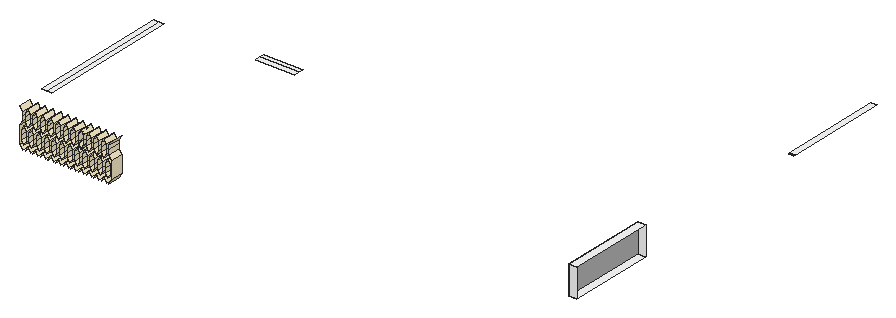
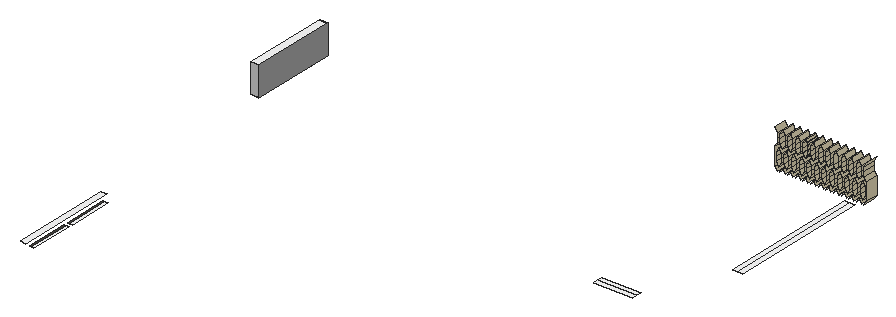
# SketchUp Ruby script. Lengths in inches.
U = 1.inch
M = Sketchup.active_model
def pt(a) = Geom::Point3d.new(a.map { |v| v * U })
def face(e, loops, mat)
  f = e.add_face(loops[0].map { |a| pt(a) })
  loops[1..].each { |l| e.add_face(l.map { |a| pt(a) }).erase! }
  f.material = f.back_material = mat if mat
  f
end
# faces: each face lists its corners as indices into pts; further lists are holes
def faces(e, pts, list, mat = nil) = list.each { |f| face(e, (f[0].is_a?(Array) ? f : [f]).map { |l| l.map { |i| pts[i] } }, mat) }
# xy, xz, yz: faces in a plane at the given z, y or x. An outline is a flat list of corners, or four numbers for a rectangle; further outlines are holes
def ring(l) = l.size == 4 ? [[l[0], l[1]], [l[2], l[1]], [l[2], l[3]], [l[0], l[3]]] : l.each_slice(2).to_a
def flat(e, list, mat, &to3) = list.each { |f| face(e, (f[0].is_a?(Array) ? f : [f]).map { |l| ring(l).map { |u, v| to3.(u, v) } }, mat) }
def xy(e, z, list, mat = nil) = flat(e, list, mat) { |x, y| [x, y, z] }
def xz(e, y, list, mat = nil) = flat(e, list, mat) { |x, z| [x, y, z] }
def yz(e, x, list, mat = nil) = flat(e, list, mat) { |y, z| [x, y, z] }
def lines(e, pts, list) = list.each { |a, b| e.add_line(pt(pts[a]), pt(pts[b])) }
# prism: a flat outline (further loops are holes) pulled along v
def prism(e, loops, v, mat = nil)
  f = face(e, loops, mat); d = Geom::Vector3d.new(v.map { |x| x * U })
  f.pushpull(f.normal.samedirection?(d) ? d.length : -d.length)
end
def box(e, o, s, mat = nil) = prism(e, [[o, [o[0] + s[0], o[1], o[2]], [o[0] + s[0], o[1] + s[1], o[2]], [o[0], o[1] + s[1], o[2]]]], [0, 0, s[2]], mat)
def at(x, y, z, deg = 0) = Geom::Transformation.translation(pt([x, y, z])) * Geom::Transformation.rotation(ORIGIN, Z_AXIS, deg.degrees)
def axes(o, x, y, z) = Geom::Transformation.new([*x, 0, *y, 0, *z, 0, *pt(o).to_a, 1])
def part(name) = M.definitions.add(name)
# library, detail: a bought-in or finely detailed component or shape, given as its bounding box
def library(name, o, s) = part(name).tap { |d| box(d.entities, o, s) }
def detail(e, o, s) = box(e.add_group.entities, o, s)
def put(e, d, t, mat = nil) = e.add_instance(d, t).tap { |i| i.material = mat if mat }
def group(e, t, mat = nil) = e.add_group.tap { |g| g.transformation = t; g.material = mat if mat }.entities
root = M.entities
M.materials.add("D01_Frost_White").color = [255, 242, 206]
M.materials.add("Glass_Mirror_01").color = [185, 185, 185]
M.materials.add("M00_Soft_Cloud").color = [255, 255, 255]
M.materials.add("Wood_Planks_01_1K").color = [69, 67, 63]
xy(root,220.1287,[[555,437.068,557.1509,475.3136],[555,479.3136,557.1509,517.5592]],"M00_Soft_Cloud")
xy(root,220.1287,[[557.1509,437.068,559.3018,475.3136],[557.1509,479.3136,559.3018,517.5592]],"Wood_Planks_01_1K")
xy(root,221.934,[[189.7692,309,223.7462,313.5],[189.7692,313.5,223.7462,318]],"M00_Soft_Cloud")
xy(root,222.3305,[[564,184.6361,571,259.8187]],"M00_Soft_Cloud")
xy(root,224.1287,[[559.3018,433.068,564,521.5592]],"M00_Soft_Cloud")
xy(root,242.0154,[[196.5333,109.0676,196.5333,109.0676,196.5333,119.6039,196.5333,119.6039]],"D01_Frost_White")
xy(root,245.0192,[[126,153.6841,130.5,276.2837],[130.5,153.6841,135,276.2837]],"M00_Soft_Cloud")
xy(root,247.6528,[[564,184.6361,571,259.8187]],"M00_Soft_Cloud")
xy(root,253.2819,[[194.3471,109.0676,194.3471,109.0676,194.3471,119.6039,194.3471,119.6039]],"D01_Frost_White")
xz(root,109.0676,[[209.933,226.9934,209.933,227.0116,209.9276,227.0025],[196.5368,242.0094,196.5404,242.0154,196.5368,242.0215,196.5333,242.0154],[209.933,242.0094,209.933,242.0154,209.9312,242.0124],[183.1639,242.0124,183.1675,242.0185,183.1639,242.0245],[196.5333,242.0154,196.5333,242.0154,196.5261,242.0276],
  [196.5333,242.0154,196.5368,242.0215,196.5297,242.0336,196.5261,242.0276],[196.5404,242.0154,198.7337,245.7225,196.5368,242.0215],[196.5368,242.0215,198.7337,245.7225,196.5297,242.0336],[169.7802,242.0276,167.5797,245.7709,167.5797,245.7831],[196.5261,242.0276,195.801,243.2733,195.4366,243.8932],
  [196.5261,242.0276,196.0916,242.7789,195.801,243.2733],[196.5261,242.0276,196.5297,242.0336,196.0916,242.7789],[196.0916,242.7789,194.3399,245.8073,194.3399,245.783,195.801,243.2733],[195.4366,243.8932,194.3399,245.7709,194.3399,245.7588],[198.7337,245.7225,198.7409,245.7345,198.7409,245.7345],
  [198.7337,245.7225,198.7409,245.7345,198.7516,253.203],[198.7409,245.7345,198.7409,245.7345,198.7444,245.7406],[198.7409,245.7345,198.7444,245.7406,198.7516,253.203],[198.7444,245.7406,198.7552,245.7588,198.7552,253.2576,196.5547,257.001,196.5618,256.9888,198.7516,253.2394,198.7516,253.203],[194.3399,245.7709,194.3399,245.783,194.3364,245.7891,194.3363,245.777],
  [194.3399,245.783,194.3399,245.8073,194.3364,245.8134,194.3364,245.7891],[167.5797,245.7831,167.5797,253.2698,167.5833,253.2759],[194.3364,245.7891,194.3364,245.8134,194.3363,245.7892],[194.3399,245.8073,194.3399,247.2979,194.3364,245.8134],[194.3364,245.8134,194.3399,247.2979,194.3399,248.2868],
  [194.3364,245.8134,194.3399,248.2868,194.3399,249.5264],[194.3399,247.2979,194.3542,253.2819,194.347,253.2698,194.3435,253.2637,194.3435,253.2759,194.3471,253.2819,194.347,253.2698,194.3399,248.2868],[194.3399,249.5264,194.3435,253.2637,194.3399,253.2576],[198.7516,253.203,198.7516,253.2273,196.5618,256.9888],[198.7516,253.203,198.7516,253.2273,198.7516,253.2273],
  [198.7516,253.2273,198.7516,253.2394,196.5618,256.9888],[194.3435,253.2637,194.347,253.2698,194.3471,253.2819,194.3435,253.2759],[194.347,253.2698,194.3542,253.2819,194.3542,253.294,194.3471,253.2819],[194.3471,253.2819,194.3471,253.2819,194.3542,253.294],[194.3542,253.2819,194.7923,254.0272,194.3542,253.294],
  [194.3542,253.294,194.7923,254.0272,195.0829,254.5216],[194.3542,253.294,195.0829,254.5216,195.4473,255.1415],[194.7923,254.0272,196.5618,256.9888,196.5547,257.001,195.0829,254.5216],[195.0829,254.5216,196.5547,257.001,196.5529,257.004,196.5493,257.004,195.4473,255.1415],[195.4473,255.1415,196.5493,257.004,196.5422,257.004]],"D01_Frost_White")
xz(root,184.6361,[[564,222.3305,571,247.6528]],"M00_Soft_Cloud")
xz(root,259.8187,[[564,222.3305,571,247.6528]],"M00_Soft_Cloud")
yz(root,143.0236,[[109.0676,227.0238,119.6039,242.0215]],"D01_Frost_White")
yz(root,144.165,[[109.0676,230.7732,119.6039,234.5226],[109.0676,234.5226,119.6039,238.2721]],"D01_Frost_White")
yz(root,145.2277,[[109.0676,245.7709,119.6039,249.5204],[109.0676,249.5204,119.6039,253.2698]],"D01_Frost_White")
yz(root,147.5105,[[109.0676,245.7709,119.6039,249.5204],[109.0676,249.5204,119.6039,253.2698]],"D01_Frost_White")
yz(root,148.5731,[[109.0676,230.7732,119.6039,234.5226],[109.0676,234.5226,119.6039,238.2721]],"D01_Frost_White")
yz(root,150.856,[[109.0676,230.7732,119.6039,234.5226],[109.0676,234.5226,119.6039,238.2721]],"D01_Frost_White")
yz(root,151.9186,[[109.0676,245.7709,119.6039,249.5204],[109.0676,249.5204,119.6039,253.2698]],"D01_Frost_White")
yz(root,154.2015,[[109.0676,245.7709,119.6039,249.5204],[109.0676,249.5204,119.6039,253.2698]],"D01_Frost_White")
yz(root,155.2641,[[109.0676,230.7732,119.6039,234.5226],[109.0676,234.5226,119.6039,238.2721]],"D01_Frost_White")
yz(root,157.5433,[[109.0676,230.7732,119.6039,234.5226],[109.0676,234.5226,119.6039,238.2721]],"D01_Frost_White")
yz(root,158.606,[[109.0676,245.7709,119.6039,249.5204],[109.0676,249.5204,119.6039,253.2698]],"D01_Frost_White")
yz(root,160.8888,[[109.0676,245.7709,119.6039,249.5204],[109.0676,249.5204,119.6039,253.2698]],"D01_Frost_White")
yz(root,161.9514,[[109.0676,230.7732,119.6039,234.5226],[109.0676,234.5226,119.6039,238.2721]],"D01_Frost_White")
yz(root,164.2343,[[109.0676,230.7732,119.6039,234.5226],[109.0676,234.5226,119.6039,238.2721]],"D01_Frost_White")
yz(root,165.2969,[[109.0676,245.7709,119.6039,249.5204],[109.0676,249.5204,119.6039,253.2698]],"D01_Frost_White")
yz(root,167.5797,[[109.0676,245.7709,119.6039,245.7831],[109.0676,245.7831,119.6039,249.5204],[109.0676,249.5204,119.6039,253.2698]],"D01_Frost_White")
yz(root,168.6424,[[109.0676,230.7732,119.6039,234.5226],[109.0676,234.5226,119.6039,238.2721]],"D01_Frost_White")
yz(root,170.9288,[[109.0676,230.7671,119.6039,234.5166],[109.0676,234.5166,119.6039,238.266]],"D01_Frost_White")
yz(root,174.2743,[[109.0676,245.7649,119.6039,249.5143],[109.0676,249.5143,119.6039,253.2637]],"D01_Frost_White")
yz(root,175.3369,[[109.0676,230.7671,119.6039,234.5166],[109.0676,234.5166,119.6039,238.266]],"D01_Frost_White")
yz(root,177.6197,[[109.0676,230.7671,119.6039,234.5166],[109.0676,234.5166,119.6039,238.266]],"D01_Frost_White")
yz(root,178.6824,[[109.0676,245.7649,119.6039,249.5143],[109.0676,249.5143,119.6039,253.2637]],"D01_Frost_White")
yz(root,180.9652,[[109.0676,245.7649,119.6039,249.5143],[109.0676,249.5143,119.6039,253.2637]],"D01_Frost_White")
yz(root,182.0278,[[109.0676,230.7671,119.6039,234.5166],[109.0676,234.5166,119.6039,238.266]],"D01_Frost_White")
yz(root,183.1639,[[109.0676,242.0124,119.6039,242.0245]],"D01_Frost_White")
yz(root,184.3035,[[109.0676,230.7611,119.6039,234.5105],[109.0676,234.5105,119.6039,238.2599]],"D01_Frost_White")
yz(root,185.3661,[[109.0676,245.7588,119.6039,249.5082],[109.0676,249.5082,119.6039,253.2576]],"D01_Frost_White")
yz(root,187.649,[[109.0676,245.7588,119.6039,249.5082],[109.0676,249.5082,119.6039,253.2576]],"D01_Frost_White")
yz(root,188.7116,[[109.0676,230.7611,119.6039,234.5105],[109.0676,234.5105,119.6039,238.2599]],"D01_Frost_White")
yz(root,190.9945,[[109.0676,230.7611,119.6039,234.5105],[109.0676,234.5105,119.6039,238.2599]],"D01_Frost_White")
yz(root,192.0571,[[109.0676,245.7588,119.6039,249.5082],[109.0676,249.5082,119.6039,253.2576]],"D01_Frost_White")
yz(root,194.3399,[[109.0676,245.7588,119.6039,245.7709],[109.0676,245.7709,119.6039,245.783],[109.0676,245.783,119.6039,245.8073],[109.0676,247.2979,119.6039,248.2868],[109.0676,248.2868,119.6039,249.5082],
  [109.0676,249.5082,119.6039,249.5264],[109.0676,249.5264,119.6039,253.2576]],"D01_Frost_White")
yz(root,194.3435,[[109.0676,253.2637,119.6039,253.2759]],"D01_Frost_White")
yz(root,194.3542,[[109.0676,253.2819,119.6039,253.294]],"D01_Frost_White")
yz(root,195.4025,[[109.0676,230.7611,119.6039,234.5105],[109.0676,234.5105,119.6039,238.2599]],"D01_Frost_White")
yz(root,197.6925,[[109.0676,230.7611,119.6039,234.5105],[109.0676,234.5105,119.6039,238.2599]],"D01_Frost_White")
yz(root,198.7552,[[109.0676,245.7588,119.6039,249.5082],[109.0676,249.5082,119.6039,253.2576]],"D01_Frost_White")
yz(root,201.038,[[109.0676,245.7588,119.6039,249.5082],[109.0676,249.5082,119.6039,253.2576]],"D01_Frost_White")
yz(root,202.1006,[[109.0676,230.7611,119.6039,234.5105],[109.0676,234.5105,119.6039,238.2599]],"D01_Frost_White")
yz(root,204.3835,[[109.0676,230.7611,119.6039,234.5105],[109.0676,234.5105,119.6039,238.2599]],"D01_Frost_White")
yz(root,205.4461,[[109.0676,245.7588,119.6039,249.5082],[109.0676,249.5082,119.6039,253.2576]],"D01_Frost_White")
yz(root,207.7289,[[109.0676,245.7588,119.6039,249.5082],[109.0676,249.5082,119.6039,253.2576]],"D01_Frost_White")
yz(root,208.7916,[[109.0676,230.7611,119.6039,234.5105],[109.0676,234.5105,119.6039,238.2599]],"D01_Frost_White")
yz(root,209.933,[[109.0676,226.9934,119.6039,227.0116],[109.0676,242.0094,119.6039,242.0154]],"D01_Frost_White")
yz(root,211.0673,[[109.0676,230.755,119.6039,234.5044],[109.0676,234.5044,119.6039,238.2539]],"D01_Frost_White")
yz(root,212.1299,[[109.0676,245.7527,119.6039,249.5021],[109.0676,249.5021,119.6039,253.2516]],"D01_Frost_White")
yz(root,214.4127,[[109.0676,245.7527,119.6039,249.5021],[109.0676,249.5021,119.6039,253.2516]],"D01_Frost_White")
yz(root,215.4754,[[109.0676,230.755,119.6039,234.5044],[109.0676,234.5044,119.6039,238.2539]],"D01_Frost_White")
yz(root,217.7582,[[109.0676,230.755,119.6039,234.5044],[109.0676,234.5044,119.6039,238.2539]],"D01_Frost_White")
yz(root,218.8208,[[109.0676,245.7527,119.6039,249.5021],[109.0676,249.5021,119.6039,253.2516]],"D01_Frost_White")
yz(root,221.1037,[[109.0676,245.7527,119.6039,249.5021],[109.0676,249.5021,119.6039,253.2516]],"D01_Frost_White")
yz(root,222.1663,[[109.0676,230.755,119.6039,234.5044],[109.0676,234.5044,119.6039,238.2539]],"D01_Frost_White")
yz(root,223.3077,[[109.0676,227.0056,119.6039,242.0033]],"D01_Frost_White")
yz(root,564,[[184.6361,222.3305,259.8187,247.6528]],"Glass_Mirror_01")
p = [[143.0236,109.0676,227.0238],[145.2277,109.0676,223.2743],[145.2277,119.6039,223.2743],[143.0236,119.6039,227.0238],[147.5105,109.0676,223.2743],[149.7146,109.0676,227.0238],
  [149.7146,119.6039,227.0238],[147.5105,119.6039,223.2743],[151.9186,109.0676,223.2743],[151.9186,119.6039,223.2743],[154.2015,109.0676,223.2743],[156.4037,109.0676,227.0207],
  [156.4037,119.6039,227.0207],[154.2015,119.6039,223.2743],[158.606,109.0676,223.2743],[158.606,119.6039,223.2743],[160.8888,109.0676,223.2743],[163.0929,109.0676,227.0238],
  [163.0929,119.6039,227.0238],[160.8888,119.6039,223.2743],[165.2969,109.0676,223.2743],[165.2969,119.6039,223.2743],[167.5797,109.0676,223.2743],[167.5833,109.0676,223.2804],
  [167.5833,119.6039,223.2804],[167.5797,119.6039,223.2743],[169.7874,109.0676,227.0177],[169.7874,119.6039,227.0177],[171.9878,109.0676,223.2622],[171.9878,119.6039,223.2622],
  [174.2743,109.0676,223.2683],[176.4783,109.0676,227.0177],[176.4783,119.6039,227.0177],[174.2743,119.6039,223.2683],[178.6824,109.0676,223.2683],[178.6824,119.6039,223.2683],
  [180.9652,109.0676,223.2683],[183.1639,109.0676,227.0086],[183.1639,119.6039,227.0086],[180.9652,119.6039,223.2683],[185.3661,109.0676,223.2622],[185.3661,119.6039,223.2622],
  [187.649,109.0676,223.2622],[189.853,109.0676,227.0116],[189.853,119.6039,227.0116],[187.649,119.6039,223.2622],[192.0571,109.0676,223.2622],[192.0571,119.6039,223.2622],
  [194.3399,109.0676,223.2622],[196.544,109.0676,227.0116],[196.544,119.6039,227.0116],[194.3399,119.6039,223.2622],[198.748,109.0676,223.2622],[198.748,119.6039,223.2622],
  [201.038,109.0676,223.2622],[203.242,109.0676,227.0116],[203.242,119.6039,227.0116],[201.038,119.6039,223.2622],[205.4461,109.0676,223.2622],[205.4461,119.6039,223.2622],
  [207.7289,109.0676,223.2622],[209.9276,109.0676,227.0025],[209.9276,119.6039,227.0025],[207.7289,119.6039,223.2622],[209.933,109.0676,226.9934],[212.1299,109.0676,223.2561],
  [212.1299,119.6039,223.2561],[209.933,119.6039,226.9934],[214.4127,109.0676,223.2561],[216.6168,109.0676,227.0056],[216.6168,119.6039,227.0056],[214.4127,119.6039,223.2561],
  [218.8208,109.0676,223.2561],[218.8208,119.6039,223.2561],[221.1037,109.0676,223.2561],[223.3077,109.0676,227.0056],[223.3077,119.6039,227.0056],[221.1037,119.6039,223.2561],
  [146.3691,109.0676,227.0238],[144.165,109.0676,230.7732],[144.165,119.6039,230.7732],[146.3691,119.6039,227.0238],[148.5731,109.0676,230.7732],[148.5731,119.6039,230.7732],
  [153.06,109.0676,227.0238],[150.856,109.0676,230.7732],[150.856,119.6039,230.7732],[153.06,119.6039,227.0238],[155.2641,109.0676,230.7732],[155.2641,119.6039,230.7732],
  [159.7474,109.0676,227.0238],[157.5433,109.0676,230.7732],[157.5433,119.6039,230.7732],[159.7474,119.6039,227.0238],[161.9514,109.0676,230.7732],[161.9514,119.6039,230.7732],
  [166.4383,109.0676,227.0238],[164.2343,109.0676,230.7732],[164.2343,119.6039,230.7732],[166.4383,119.6039,227.0238],[168.6424,109.0676,230.7732],[168.6424,119.6039,230.7732],
  [173.1328,109.0676,227.0177],[170.9288,109.0676,230.7671],[170.9288,119.6039,230.7671],[173.1328,119.6039,227.0177],[175.3369,109.0676,230.7671],[175.3369,119.6039,230.7671],
  [179.8238,109.0676,227.0177],[177.6197,109.0676,230.7671],[177.6197,119.6039,230.7671],[179.8238,119.6039,227.0177],[182.0278,109.0676,230.7671],[182.0278,119.6039,230.7671],
  [186.5076,109.0676,227.0116],[184.3035,109.0676,230.7611],[184.3035,119.6039,230.7611],[186.5076,119.6039,227.0116],[188.7116,109.0676,230.7611],[188.7116,119.6039,230.7611],
  [193.1985,109.0676,227.0116],[190.9945,109.0676,230.7611],[190.9945,119.6039,230.7611],[193.1985,119.6039,227.0116],[195.4025,109.0676,230.7611],[195.4025,119.6039,230.7611],
  [199.8966,109.0676,227.0116],[197.6925,109.0676,230.7611],[197.6925,119.6039,230.7611],[199.8966,119.6039,227.0116],[202.1006,109.0676,230.7611],[202.1006,119.6039,230.7611],
  [206.5875,109.0676,227.0116],[204.3835,109.0676,230.7611],[204.3835,119.6039,230.7611],[206.5875,119.6039,227.0116],[208.7916,109.0676,230.7611],[208.7916,119.6039,230.7611],
  [209.933,109.0676,227.0116],[209.933,119.6039,227.0116],[213.2713,109.0676,227.0056],[211.0673,109.0676,230.755],[211.0673,119.6039,230.755],[213.2713,119.6039,227.0056],
  [215.4754,109.0676,230.755],[215.4754,119.6039,230.755],[219.9622,109.0676,227.0056],[217.7582,109.0676,230.755],[217.7582,119.6039,230.755],[219.9622,119.6039,227.0056],
  [222.1663,109.0676,230.755],[222.1663,119.6039,230.755],[144.165,109.0676,238.2721],[146.3691,109.0676,242.0215],[146.3691,119.6039,242.0215],[144.165,119.6039,238.2721],
  [148.5731,109.0676,238.2721],[148.5731,119.6039,238.2721],[150.856,109.0676,238.2721],[153.06,109.0676,242.0215],[153.06,119.6039,242.0215],[150.856,119.6039,238.2721],
  [155.2641,109.0676,238.2721],[155.2641,119.6039,238.2721],[157.5433,109.0676,238.2721],[159.7474,109.0676,242.0215],[159.7474,119.6039,242.0215],[157.5433,119.6039,238.2721],
  [161.9514,109.0676,238.2721],[161.9514,119.6039,238.2721],[164.2343,109.0676,238.2721],[166.4383,109.0676,242.0215],[166.4383,119.6039,242.0215],[164.2343,119.6039,238.2721],
  [168.6424,109.0676,238.2721],[168.6424,119.6039,238.2721],[170.9288,109.0676,238.266],[173.1328,109.0676,242.0154],[173.1328,119.6039,242.0154],[170.9288,119.6039,238.266],
  [175.3369,109.0676,238.266],[175.3369,119.6039,238.266],[177.6197,109.0676,238.266],[179.8238,109.0676,242.0154],[179.8238,119.6039,242.0154],[177.6197,119.6039,238.266],
  [182.0278,109.0676,238.266],[182.0278,119.6039,238.266],[184.3035,109.0676,238.2599],[186.5076,109.0676,242.0094],[186.5076,119.6039,242.0094],[184.3035,119.6039,238.2599],
  [188.7116,109.0676,238.2599],[188.7116,119.6039,238.2599],[190.9945,109.0676,238.2599],[193.1985,109.0676,242.0094],[193.1985,119.6039,242.0094],[190.9945,119.6039,238.2599],
  [195.4025,109.0676,238.2599],[195.4025,119.6039,238.2599],[197.6925,109.0676,238.2599],[199.8966,109.0676,242.0094],[199.8966,119.6039,242.0094],[197.6925,119.6039,238.2599],
  [202.1006,109.0676,238.2599],[202.1006,119.6039,238.2599],[204.3835,109.0676,238.2599],[206.5875,109.0676,242.0094],[206.5875,119.6039,242.0094],[204.3835,119.6039,238.2599],
  [208.7916,109.0676,238.2599],[208.7916,119.6039,238.2599],[211.0673,109.0676,238.2539],[213.2713,109.0676,242.0033],[213.2713,119.6039,242.0033],[211.0673,119.6039,238.2539],
  [215.4754,109.0676,238.2539],[215.4754,119.6039,238.2539],[217.7582,109.0676,238.2539],[219.9622,109.0676,242.0033],[219.9622,119.6039,242.0033],[217.7582,119.6039,238.2539],
  [222.1663,109.0676,238.2539],[222.1663,119.6039,238.2539],[145.2277,109.0676,245.7709],[143.0236,109.0676,242.0215],[143.0236,119.6039,242.0215],[145.2277,119.6039,245.7709],
  [149.7146,109.0676,242.0215],[147.5105,109.0676,245.7709],[147.5105,119.6039,245.7709],[149.7146,119.6039,242.0215],[151.9186,109.0676,245.7709],[151.9186,119.6039,245.7709],
  [156.4037,109.0676,242.0245],[154.2015,109.0676,245.7709],[154.2015,119.6039,245.7709],[156.4037,119.6039,242.0245],[158.606,109.0676,245.7709],[158.606,119.6039,245.7709],
  [163.0929,109.0676,242.0215],[160.8888,109.0676,245.7709],[160.8888,119.6039,245.7709],[163.0929,119.6039,242.0215],[165.2969,109.0676,245.7709],[165.2969,119.6039,245.7709],
  [169.7802,109.0676,242.0276],[167.5797,109.0676,245.7709],[167.5797,119.6039,245.7709],[169.7802,119.6039,242.0276],[171.9843,109.0676,245.7649],[171.9843,119.6039,245.7649],
  [176.4783,109.0676,242.0154],[174.2743,109.0676,245.7649],[174.2743,119.6039,245.7649],[176.4783,119.6039,242.0154],[178.6824,109.0676,245.7649],[178.6824,119.6039,245.7649],
  [183.1639,109.0676,242.0245],[180.9652,109.0676,245.7649],[180.9652,119.6039,245.7649],[183.1639,119.6039,242.0245],[183.1675,109.0676,242.0185],[183.1639,109.0676,242.0124],
  [183.1639,119.6039,242.0124],[183.1675,119.6039,242.0185],[185.3661,109.0676,245.7588],[185.3661,119.6039,245.7588],[189.853,109.0676,242.0094],[187.649,109.0676,245.7588],
  [187.649,119.6039,245.7588],[189.853,119.6039,242.0094],[192.0571,109.0676,245.7588],[192.0571,119.6039,245.7588],[196.5261,109.0676,242.0276],[195.4366,109.0676,243.8932],
  [195.4366,119.6039,243.8932],[196.5261,119.6039,242.0276],[196.5404,109.0676,242.0154],[196.5368,109.0676,242.0094],[196.5368,119.6039,242.0094],[196.5404,119.6039,242.0154],
  [196.5333,109.0676,242.0154],[196.5333,119.6039,242.0154],[196.5368,109.0676,242.0215],[196.5368,119.6039,242.0215],[196.5333,109.0676,242.0154],[196.5333,119.6039,242.0154],
  [198.7337,109.0676,245.7225],[198.7337,119.6039,245.7225],[203.242,109.0676,242.0094],[201.038,109.0676,245.7588],[201.038,119.6039,245.7588],[203.242,119.6039,242.0094],
  [205.4461,109.0676,245.7588],[205.4461,119.6039,245.7588],[209.9312,109.0676,242.0124],[207.7289,109.0676,245.7588],[207.7289,119.6039,245.7588],[209.9312,119.6039,242.0124],
  [209.933,109.0676,242.0094],[209.933,119.6039,242.0094],[212.1299,109.0676,245.7527],[209.933,109.0676,242.0154],[209.933,119.6039,242.0154],[212.1299,119.6039,245.7527],
  [216.6168,109.0676,242.0033],[214.4127,109.0676,245.7527],[214.4127,119.6039,245.7527],[216.6168,119.6039,242.0033],[218.8208,109.0676,245.7527],[218.8208,119.6039,245.7527],
  [223.3077,109.0676,242.0033],[221.1037,109.0676,245.7527],[221.1037,119.6039,245.7527],[223.3077,119.6039,242.0033],[196.0916,109.0676,242.7789],[194.3399,109.0676,245.8073],
  [194.3399,119.6039,245.8073],[196.0916,119.6039,242.7789],[195.801,109.0676,243.2733],[195.801,119.6039,243.2733],[194.3399,109.0676,245.7709],[194.3399,119.6039,245.7709],
  [194.3399,109.0676,245.7588],[194.3399,119.6039,245.7588],[198.7409,109.0676,245.7345],[198.7409,119.6039,245.7345],[198.7444,109.0676,245.7406],[198.7444,119.6039,245.7406],
  [198.7552,109.0676,245.7588],[198.7552,119.6039,245.7588],[171.9878,109.0676,253.2576],[171.9878,119.6039,253.2576],[194.3363,109.0676,245.777],[194.3363,119.6039,245.777],
  [194.3364,109.0676,245.7891],[194.3364,119.6039,245.7891],[194.3363,109.0676,245.7892],[194.3363,119.6039,245.7892],[194.3364,109.0676,245.8134],[194.3364,119.6039,245.8134],
  [194.3399,109.0676,249.5264],[194.3399,119.6039,249.5264],[194.3399,109.0676,247.2979],[194.3542,109.0676,253.2819],[194.3542,119.6039,253.2819],[194.3399,119.6039,247.2979],
  [194.3435,109.0676,253.2637],[194.3435,119.6039,253.2637],[143.0236,109.0676,257.0192],[145.2277,109.0676,253.2698],[145.2277,119.6039,253.2698],[143.0236,119.6039,257.0192],
  [147.5105,109.0676,253.2698],[149.7146,109.0676,257.0192],[149.7146,119.6039,257.0192],[147.5105,119.6039,253.2698],[151.9186,109.0676,253.2698],[151.9186,119.6039,253.2698],
  [154.2015,109.0676,253.2698],[156.4037,109.0676,257.0162],[156.4037,119.6039,257.0162],[154.2015,119.6039,253.2698],[158.606,109.0676,253.2698],[158.606,119.6039,253.2698],
  [160.8888,109.0676,253.2698],[163.0929,109.0676,257.0192],[163.0929,119.6039,257.0192],[160.8888,119.6039,253.2698],[165.2969,109.0676,253.2698],[165.2969,119.6039,253.2698],
  [167.5797,109.0676,253.2698],[167.5833,109.0676,253.2759],[167.5833,119.6039,253.2759],[167.5797,119.6039,253.2698],[169.7838,109.0676,257.0192],[169.7838,119.6039,257.0192],
  [169.7874,109.0676,257.0132],[169.7874,119.6039,257.0132],[174.2743,109.0676,253.2637],[176.4783,109.0676,257.0132],[176.4783,119.6039,257.0132],[174.2743,119.6039,253.2637],
  [178.6824,109.0676,253.2637],[178.6824,119.6039,253.2637],[180.9652,109.0676,253.2637],[183.1639,109.0676,257.004],[183.1639,119.6039,257.004],[180.9652,119.6039,253.2637],
  [185.3661,109.0676,253.2576],[185.3661,119.6039,253.2576],[187.649,109.0676,253.2576],[189.8512,109.0676,257.004],[189.8512,119.6039,257.004],[187.649,119.6039,253.2576],
  [189.8548,109.0676,257.004],[192.0571,109.0676,253.2576],[192.0571,119.6039,253.2576],[189.8548,119.6039,257.004],[194.3399,109.0676,253.2576],[194.3399,119.6039,253.2576],
  [194.347,109.0676,253.2698],[194.347,119.6039,253.2698],[194.3471,109.0676,253.2819],[194.3471,119.6039,253.2819],[194.3435,109.0676,253.2759],[194.3435,119.6039,253.2759],
  [194.3542,109.0676,253.294],[194.3542,119.6039,253.294],[194.3471,109.0676,253.2819],[194.3471,119.6039,253.2819],[195.0829,109.0676,254.5216],[195.0829,119.6039,254.5216],
  [196.5547,109.0676,257.001],[198.7552,109.0676,253.2576],[198.7552,119.6039,253.2576],[196.5547,119.6039,257.001],[201.038,109.0676,253.2576],[203.242,109.0676,257.0071],
  [203.242,119.6039,257.0071],[201.038,119.6039,253.2576],[205.4461,109.0676,253.2576],[205.4461,119.6039,253.2576],[207.7289,109.0676,253.2576],[209.9276,109.0676,256.998],
  [209.9276,119.6039,256.998],[207.7289,119.6039,253.2576],[209.933,109.0676,256.9889],[212.1299,109.0676,253.2516],[212.1299,119.6039,253.2516],[209.933,119.6039,256.9889],
  [214.4127,109.0676,253.2516],[216.6168,109.0676,257.001],[216.6168,119.6039,257.001],[214.4127,119.6039,253.2516],[218.8208,109.0676,253.2516],[218.8208,119.6039,253.2516],
  [221.1037,109.0676,253.2516],[223.3077,109.0676,257.001],[223.3077,119.6039,257.001],[221.1037,119.6039,253.2516],[195.4473,109.0676,255.1415],[195.4473,119.6039,255.1415],
  [196.5422,109.0676,257.004],[196.5422,119.6039,257.004],[196.544,109.0676,242.0094],[183.1692,109.0676,227.0177],[169.7838,109.0676,227.0238],[198.7409,109.0676,245.7345],
  [196.5547,109.0676,242.0154],[183.1621,109.0676,227.0116],[156.4055,109.0676,242.0215],[156.4019,109.0676,242.0215],[183.1621,109.0676,242.0094],[183.1692,109.0676,242.0154],
  [171.9914,109.0676,253.2637],[171.9914,109.0676,249.5143],[171.9914,109.0676,245.7649],[169.7874,109.0676,242.0154],[171.9914,109.0676,223.2683],[209.9276,109.0676,242.0063],
  [209.9258,109.0676,242.0033],[196.5511,109.0676,242.0094],[156.4019,109.0676,227.0238],[156.4055,109.0676,227.0238],[169.7838,109.0676,242.0215],[209.9258,109.0676,227.0056]]
faces(root,p,[[0,1,2,3],[4,5,6,7],[5,8,9,6],[10,11,12,13],[11,14,15,12],[16,17,18,19],[17,20,21,18],[22,23,24,25],
  [23,26,27,24],[26,28,29,27],[30,31,32,33],[31,34,35,32],[36,37,38,39],[37,40,41,38],[42,43,44,45],[43,46,47,44],
  [48,49,50,51],[49,52,53,50],[54,55,56,57],[55,58,59,56],[60,61,62,63],[64,65,66,67],[68,69,70,71],[69,72,73,70],
  [74,75,76,77],[78,79,80,81],[82,78,81,83],[84,85,86,87],[88,84,87,89],[90,91,92,93],[94,90,93,95],[96,97,98,99],
  [100,96,99,101],[102,103,104,105],[106,102,105,107],[108,109,110,111],[112,108,111,113],[114,115,116,117],[118,114,117,119],[120,121,122,123],
  [124,120,123,125],[126,127,128,129],[130,126,129,131],[132,133,134,135],[136,132,135,137],[61,138,139,62],[140,141,142,143],[144,140,143,145],
  [146,147,148,149],[150,146,149,151],[152,153,154,155],[153,156,157,154],[158,159,160,161],[159,162,163,160],[164,165,166,167],[165,168,169,166],
  [170,171,172,173],[171,174,175,172],[176,177,178,179],[177,180,181,178],[182,183,184,185],[183,186,187,184],[188,189,190,191],[189,192,193,190],
  [194,195,196,197],[195,198,199,196],[200,201,202,203],[201,204,205,202],[206,207,208,209],[207,210,211,208],[212,213,214,215],[213,216,217,214],
  [218,219,220,221],[219,222,223,220],[224,225,226,227],[228,229,230,231],[232,228,231,233],[234,235,236,237],[238,234,237,239],[240,241,242,243],
  [244,240,243,245],[246,247,248,249],[250,246,249,251],[252,253,254,255],[256,252,255,257],[258,259,260,261],[262,263,264,265],[266,262,265,267],
  [268,269,270,271],[272,268,271,273],[274,275,276,277],[278,279,280,281],[279,282,283,280],[284,278,281,285],[286,274,277,287],[288,284,285,289],
  [290,291,292,293],[294,290,293,295],[296,297,298,299],[300,296,299,301],[302,303,304,305],[306,307,308,309],[310,306,309,311],[312,313,314,315],
  [316,317,318,319],[320,316,319,321],[275,320,321,276],[322,275,276,323],[275,324,325,276],[326,288,289,327],[328,326,327,329],[330,328,329,331],
  [332,250,251,333],[322,334,335,323],[334,336,337,335],[336,338,339,337],[338,340,341,339],[340,342,343,341],[344,345,346,347],[348,342,343,349],
  [350,351,352,353],[354,355,356,357],[355,358,359,356],[360,361,362,363],[361,364,365,362],[366,367,368,369],[367,370,371,368],[372,373,374,375],
  [373,376,377,374],[378,332,333,379],[380,381,382,383],[381,384,385,382],[386,387,388,389],[387,390,391,388],[392,393,394,395],[396,397,398,399],
  [400,348,349,401],[402,348,349,403],[404,402,403,405],[406,404,405,407],[408,404,405,409],[410,408,409,411],[408,412,413,409],[414,415,416,417],
  [418,419,420,421],[419,422,423,420],[424,425,426,427],[428,429,430,431],[432,433,434,435],[433,436,437,434],[438,439,440,441],[412,442,443,413],
  [442,444,445,443]],"D01_Frost_White")
lines(root,p,[[446,278],[37,447],[23,448],[449,450],[373,378],[451,37],[452,234],[234,453],[263,454],[455,262],[378,456],[456,457],
  [457,458],[458,459],[26,460],[461,462],[450,463],[464,11],[11,465],[466,246],[467,61],[296,461]])
